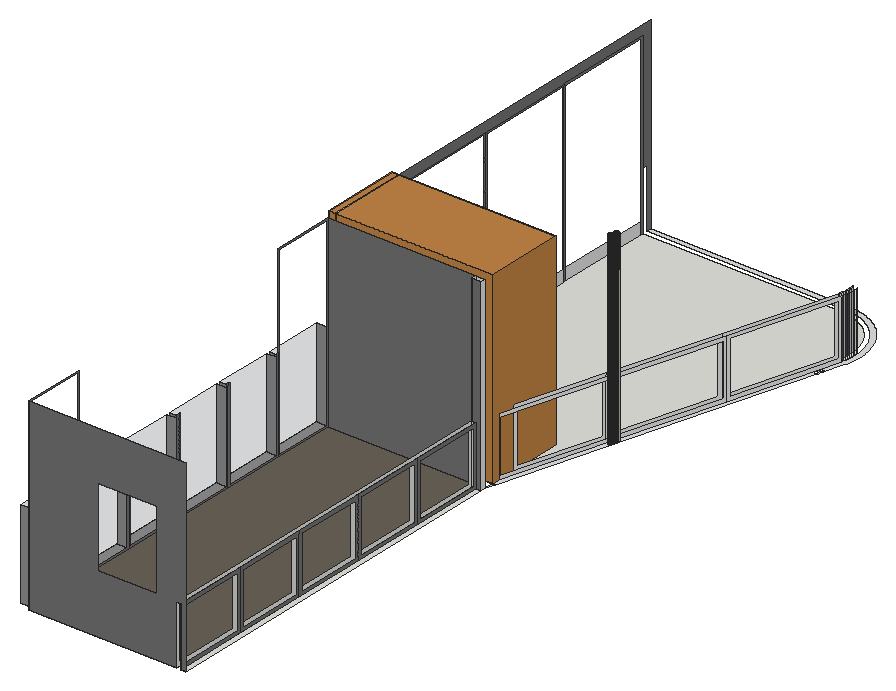
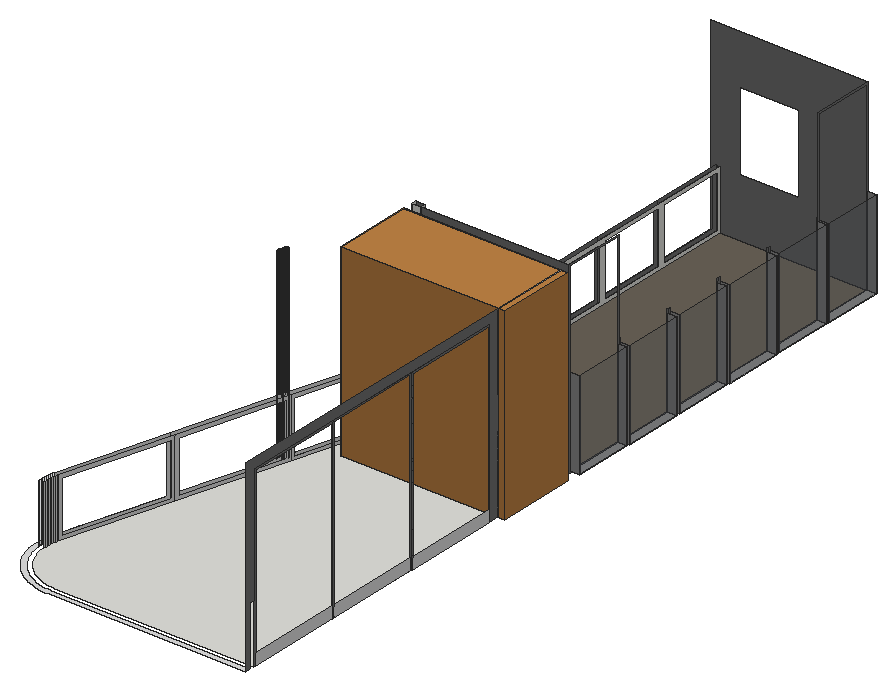
# SketchUp Ruby script. Lengths in inches.
U = 1.inch
M = Sketchup.active_model
def pt(a) = Geom::Point3d.new(a.map { |v| v * U })
def face(e, loops, mat)
  f = e.add_face(loops[0].map { |a| pt(a) })
  loops[1..].each { |l| e.add_face(l.map { |a| pt(a) }).erase! }
  f.material = f.back_material = mat if mat
  f
end
# faces: each face lists its corners as indices into pts; further lists are holes
def faces(e, pts, list, mat = nil) = list.each { |f| face(e, (f[0].is_a?(Array) ? f : [f]).map { |l| l.map { |i| pts[i] } }, mat) }
# xy, xz, yz: faces in a plane at the given z, y or x. An outline is a flat list of corners, or four numbers for a rectangle; further outlines are holes
def ring(l) = l.size == 4 ? [[l[0], l[1]], [l[2], l[1]], [l[2], l[3]], [l[0], l[3]]] : l.each_slice(2).to_a
def flat(e, list, mat, &to3) = list.each { |f| face(e, (f[0].is_a?(Array) ? f : [f]).map { |l| ring(l).map { |u, v| to3.(u, v) } }, mat) }
def xy(e, z, list, mat = nil) = flat(e, list, mat) { |x, y| [x, y, z] }
def xz(e, y, list, mat = nil) = flat(e, list, mat) { |x, z| [x, y, z] }
def yz(e, x, list, mat = nil) = flat(e, list, mat) { |y, z| [x, y, z] }
def lines(e, pts, list) = list.each { |a, b| e.add_line(pt(pts[a]), pt(pts[b])) }
# prism: a flat outline (further loops are holes) pulled along v
def prism(e, loops, v, mat = nil)
  f = face(e, loops, mat); d = Geom::Vector3d.new(v.map { |x| x * U })
  f.pushpull(f.normal.samedirection?(d) ? d.length : -d.length)
end
def box(e, o, s, mat = nil) = prism(e, [[o, [o[0] + s[0], o[1], o[2]], [o[0] + s[0], o[1] + s[1], o[2]], [o[0], o[1] + s[1], o[2]]]], [0, 0, s[2]], mat)
def at(x, y, z, deg = 0) = Geom::Transformation.translation(pt([x, y, z])) * Geom::Transformation.rotation(ORIGIN, Z_AXIS, deg.degrees)
def axes(o, x, y, z) = Geom::Transformation.new([*x, 0, *y, 0, *z, 0, *pt(o).to_a, 1])
def part(name) = M.definitions.add(name)
# library, detail: a bought-in or finely detailed component or shape, given as its bounding box
def library(name, o, s) = part(name).tap { |d| box(d.entities, o, s) }
def detail(e, o, s) = box(e.add_group.entities, o, s)
def put(e, d, t, mat = nil) = e.add_instance(d, t).tap { |i| i.material = mat if mat }
def group(e, t, mat = nil) = e.add_group.tap { |g| g.transformation = t; g.material = mat if mat }.entities
root = M.entities
M.materials.add("Glass_Basic_01").color = [105, 113, 122]
M.materials["Glass_Basic_01"].alpha = 0.25
M.materials.add("M01_Silver_Fog").color = [224, 224, 224]
M.materials.add("M04_Stone_Frost").color = [142, 142, 142]
M.materials.add("M06_Steel_Smoke").color = [114, 114, 114]
M.materials.add("Plaster_04_1K").color = [106, 98, 87]
M.materials.add("Wood_Floor_01_1K").color = [193, 132, 69]
c1 = part("Group\#1")
box(c1.entities,[-3.94,0,0],[99.94,48,114])
xy(root,396,[[303,6,306,231],[306,234,307.76,240,306,240],[216,246,303.26,246,306,255.36,321.22,307.35,340.07,371.78,359.17,437.01,359.4,437.91,359.63,439,359.83,440.1,359.98,441.21,360.09,442.32,360.16,443.43,360.1875,444.55,360.17,445.67,360.11,446.78,360.01,447.89,359.87,449,359.68,450.1,359.45,451.2,359.18,452.28,358.875,453.35,358.52,454.41,358.13,455.46,357.7,456.49,357.23,457.5,356.73,458.5,356.18,459.47,355.6,460.43,354.98,461.36,354.33,462.26,353.64,463.14,352.92,464,352.17,464.83,351.39,465.62,350.58,466.39,349.74,467.125,348.87,467.83,347.97,468.5,347.05,469.13,346.11,469.73,345.15,470.29,344.16,470.82,343.16,471.3,342.13,471.75,341.09,472.16,340.04,472.53,338.97,472.86,337.89,473.15,336.8,473.4,335.71,473.6,334.6,473.77,333.49,473.89,332.38,473.97,331.45,474,210,474,210,288,213,288,213,287.79,216,287.79]])
xy(root,396,[[[210,240,307.76,240,364.95,435.42,365.24,436.52,365.52,437.84,365.76,439.16,365.94,440.5,366.07,441.84,366.16,443.18,366.1875,444.52,366.17,445.87,366.1,447.21,365.98,448.55,365.8,449.89,365.58,451.21,365.3,452.53,364.98,453.84,364.61,455.13,364.18,456.41,363.71,457.67,363.2,458.91,362.63,460.13,362.02,461.33,361.36,462.5,360.69,463.59,360.66,463.65,359.92,464.77,359.13,465.86,358.3,466.92,357.4375,467.95,357.39,468,356.53,468.95,355.59,469.91,354.61,470.83,353.6,471.72,352.55,472.5625,351.47,473.37,350.37,474.13,349.23,474.85,348.07,475.53,346.88,476.16,345.67,476.75,344.44,477.29,343.1875,477.79,341.92,478.23,340.63,478.63,339.33,478.98,338.02,479.28,336.7,479.52,335.37,479.72,334.03,479.87,332.69,479.96,331.55,480,210,480,210,477,331.5,477,332.53,476.97,333.76,476.88,334.99,476.74,336.2,476.5625,337.41,476.34,338.61,476.0625,339.8,475.75,340.98,475.38,342.14,474.97,343.29,474.52,344.41,474.03,345.52,473.49,346.61,472.91,347.67,472.29,348.71,471.63,349.72,470.93,350.71,470.19,351.67,469.42,352.59,468.61,353.49,467.76,354.35,466.89,355.17,465.98,355.18,465.98,355.97,465.03,356.73,464.0625,357.45,463.0625,358.13,462.04,358.13,462.03,358.77,460.99,359.37,459.91,359.93,458.82,360.45,457.7,360.92,456.5625,361.35,455.41,361.74,454.24,362.08,453.06,362.38,451.86,362.63,450.66,362.83,449.44,362.99,448.22,363.1,447,363.17,445.77,363.1875,444.54,363.16,443.31,363.08,442.08,362.96,440.85,362.79,439.63,362.58,438.42,362.32,437.22,362.06,436.22,343.2,371.78,324.34,307.35,305.51,243,213,243,213,288,210,288],[358.91,418.8,358.82,418.81,358.73,418.8125,358.65,418.83,358.5625,418.85,358.48,418.87,358.39,418.9,358.3125,418.9375,358.24,418.98,358.16,419.02,358.09,419.07,357.95,419.18,357.89,419.24,357.83,419.31,357.73,419.45,357.68,419.53,357.64,419.61,357.61,419.6875,357.58,419.77,357.55,419.85,357.54,419.94,357.52,420.03,357.51,420.11,357.51,420.29,357.52,420.38,357.54,420.46,357.55,420.55,357.58,420.64,357.64,420.8,357.68,420.88,357.73,420.95,357.78,421.03,357.83,421.09,357.89,421.16,357.95,421.22,358.09,421.34,358.16,421.38,358.24,421.43,358.3125,421.47,358.39,421.5,358.48,421.53,358.5625,421.56,358.65,421.58,358.73,421.59,358.82,421.6,359,421.6,359.09,421.59,359.17,421.58,359.26,421.56,359.34,421.53,359.43,421.5,359.51,421.47,359.58,421.43,359.66,421.38,359.73,421.34,359.87,421.22,359.93,421.16,359.99,421.09,360.04,421.03,360.09,420.95,360.14,420.88,360.18,420.8,360.24,420.64,360.27,420.55,360.29,420.46,360.3,420.38,360.31,420.29,360.31,420.11,360.3,420.03,360.29,419.94,360.27,419.85,360.24,419.77,360.21,419.6875,360.18,419.61,360.14,419.53,360.09,419.45,359.99,419.31,359.93,419.24,359.87,419.18,359.73,419.07,359.66,419.02,359.58,418.98,359.51,418.9375,359.43,418.9,359.34,418.87,359.26,418.85,359.17,418.83,359.09,418.8125,359,418.81],[359.74,421.95,359.66,421.96,359.57,421.97,359.48,421.99,359.32,422.05,359.23,422.08,359.16,422.12,359.08,422.17,359.01,422.21,358.9375,422.27,358.87,422.33,358.75,422.45,358.7,422.52,358.65,422.6,358.6,422.67,358.5625,422.75,358.53,422.83,358.5,422.91,358.47,423,358.46,423.08,358.44,423.17,358.43,423.26,358.43,423.44,358.44,423.52,358.46,423.61,358.47,423.7,358.53,423.86,358.5625,423.94,358.6,424.02,358.65,424.1,358.75,424.24,358.81,424.31,358.87,424.37,358.9375,424.43,359.01,424.48,359.08,424.53,359.16,424.57,359.23,424.61,359.32,424.65,359.4,424.68,359.48,424.7,359.66,424.74,359.74,424.74,359.83,424.75,359.92,424.74,360.01,424.74,360.09,424.72,360.18,424.7,360.26,424.68,360.35,424.65,360.51,424.57,360.58,424.53,360.72,424.43,360.79,424.37,360.85,424.31,360.91,424.24,361.01,424.1,361.06,424.02,361.1,423.94,361.16,423.78,361.1875,423.7,361.21,423.61,361.22,423.52,361.23,423.44,361.23,423.26,361.21,423.08,361.1875,423,361.16,422.91,361.1,422.75,361.06,422.67,361.01,422.6,360.96,422.52,360.91,422.45,360.79,422.33,360.65,422.21,360.58,422.17,360.51,422.12,360.43,422.08,360.35,422.05,360.26,422.02,360.18,421.99,360.09,421.97,360.01,421.96,359.92,421.95],[325.27,304.17,325.18,304.18,325.09,304.1875,325.01,304.2,324.92,304.23,324.84,304.25,324.6,304.37,324.39,304.52,324.32,304.58,324.26,304.65,324.11,304.86,324.03,305.02,324,305.1,323.97,305.1875,323.95,305.27,323.9375,305.36,323.93,305.44,323.92,305.53,323.92,305.62,323.93,305.71,323.9375,305.8,323.96,305.88,323.98,305.97,324,306.05,324.12,306.29,324.27,306.5,324.33,306.56,324.4,306.625,324.47,306.68,324.61,306.78,324.77,306.86,324.85,306.89,324.9375,306.92,325.02,306.9375,325.11,306.95,325.2,306.96,325.28,306.97,325.37,306.97,325.55,306.95,325.63,306.93,325.72,306.91,325.88,306.85,325.96,306.8125,326.04,306.77,326.18,306.67,326.25,306.61,326.31,306.55,326.375,306.49,326.43,306.42,326.53,306.28,326.61,306.12,326.64,306.04,326.67,305.95,326.6875,305.87,326.7,305.78,326.71,305.69,326.72,305.61,326.72,305.52,326.7,305.34,326.68,305.26,326.66,305.17,326.6,305.01,326.5625,304.93,326.52,304.85,326.42,304.71,326.3,304.57,326.24,304.51,326.03,304.36,325.87,304.28,325.79,304.25,325.7,304.22,325.62,304.2,325.53,304.1875,325.44,304.17],[326.2,307.35,326.02,307.37,325.9375,307.38,325.85,307.41,325.77,307.43,325.6875,307.47,325.61,307.5,325.53,307.55,325.32,307.7,325.26,307.76,325.14,307.9,325.04,308.04,324.96,308.2,324.93,308.28,324.9,308.37,324.88,308.45,324.87,308.54,324.85,308.71,324.85,308.8,324.87,308.98,324.89,309.0625,324.91,309.15,324.9375,309.23,324.97,309.3125,325.01,309.39,325.05,309.47,325.2,309.68,325.27,309.74,325.33,309.8,325.4,309.86,325.54,309.96,325.7,310.04,325.78,310.07,325.87,310.1,325.95,310.12,326.04,310.13,326.21,310.15,326.3,310.15,326.48,310.13,326.5625,310.11,326.65,310.09,326.73,310.0625,326.8125,310.03,326.89,309.99,326.97,309.95,327.11,309.85,327.25,309.73,327.31,309.67,327.46,309.46,327.54,309.3,327.57,309.22,327.6,309.13,327.62,309.05,327.63,308.96,327.65,308.79,327.65,308.7,327.63,308.52,327.61,308.4375,327.59,308.35,327.56,308.27,327.53,308.1875,327.49,308.11,327.45,308.03,327.4,307.96,327.35,307.88,327.3,307.82,327.17,307.69,326.96,307.54,326.8,307.46,326.72,307.43,326.63,307.4,326.55,307.38,326.46,307.36,326.375,307.35]]],"M01_Silver_Fog")
xy(root,396,[[210,6,300,234]],"Plaster_04_1K")
xy(root,397,[[204,7,210,43],[204,45,210,81],[204,83,210,119],[204,121,210,157],[204,159,210,195],
  [204,197,210,233]],"M04_Stone_Frost")
xz(root,6,[[[210,396,210,510,306,510,306,396,303,396,303,432,300,432,300,396],[252,432,288,480]]],"M06_Steel_Smoke")
xz(root,7,[[204,397,210,451]],"M04_Stone_Frost")
xz(root,43,[[204,397,210,451]],"M04_Stone_Frost")
xz(root,45,[[204,397,210,451]],"M04_Stone_Frost")
xz(root,81,[[204,397,210,451]],"M04_Stone_Frost")
xz(root,83,[[204,397,210,451]],"M04_Stone_Frost")
xz(root,119,[[204,397,210,451]],"M04_Stone_Frost")
xz(root,121,[[204,397,210,451]],"M04_Stone_Frost")
xz(root,157,[[204,397,210,451]],"M04_Stone_Frost")
xz(root,159,[[204,397,210,451]],"M04_Stone_Frost")
xz(root,195,[[204,397,210,451]],"M04_Stone_Frost")
xz(root,197,[[204,397,210,451]],"M04_Stone_Frost")
xz(root,231,[[303,396,306,396,306,510,300,510,300,432,303,432]],"M06_Steel_Smoke")
xz(root,233,[[204,397,210,451]],"M04_Stone_Frost")
xz(root,234,[[300,396,306,510]])
xz(root,234,[[210,396,300,510]],"M06_Steel_Smoke")
xz(root,243,[[213,396,305.51,432]],"M01_Silver_Fog")
xz(root,246,[[216,396,303.26,432]],"M01_Silver_Fog")
xz(root,287.79,[[213,396,216,432]],"M01_Silver_Fog")
xz(root,304.17,[[325.27,396,325.36,510],[325.36,396,325.44,510]],"M01_Silver_Fog")
xz(root,306.97,[[325.28,396,325.37,510]],"M01_Silver_Fog")
xz(root,307.35,[[326.2,396,326.29,510],[326.29,396,326.375,510]],"M01_Silver_Fog")
xz(root,310.15,[[326.21,396,326.3,510]],"M01_Silver_Fog")
yz(root,204,[[7,397,43,451],[45,397,81,451],[83,397,119,451],[121,397,157,451],[159,397,195,451],
  [197,397,233,451]],"Glass_Basic_01")
yz(root,210,[[240,396,288,396,288,442.46,286.46,442.46,286.46,463.54,288,463.54,288,510,240,510]])
yz(root,210,[[295,396,353,403],[355,396,413,403],[415,396,473,403]],"M01_Silver_Fog")
yz(root,210,[[6,396,44,396,44,453,43,453,43,397,7,397,7,509,43,509,43,453,44,453,44,510,6,510],[44,396,82,396,82,453,81,453,81,397,45,397,45,453,44,453],[82,396,120,396,120,453,119,453,119,397,83,397,83,453,82,453],[120,396,158,396,158,453,157,453,157,397,121,397,121,453,120,453],[158,396,196,396,196,453,195,453,195,397,159,397,159,453,158,453],
  [196,396,234,396,234,510,196,510,196,453,197,453,197,509,233,509,233,397,197,397,197,453,196,453],[288,396,294,396,294,504,474,504,474,432,477,432,477,396,480,396,480,510,288,510],[294,396,295,396,295,503,353,503,353,396,354,396,354,504,294,504],[354,396,355,396,355,503,413,503,413,396,414,396,414,504,354,504],[414,396,415,396,415,503,473,503,473,396,474,396,474,504,414,504]],"M06_Steel_Smoke")
yz(root,213,[[243,396,287.79,432]],"M01_Silver_Fog")
yz(root,216,[[246,396,287.79,432]],"M01_Silver_Fog")
yz(root,300,[[[6,396,231,432],[8,398,49,430],[143,398,184,430],[188,398,229,430],[53,398,94,430],[98,398,139,430]],[231,396,234,510]])
yz(root,303,[[[6,396,51,432],[8,398,49,430]],[[51,396,96,432],[53,398,94,430]],[[96,396,141,432],[98,398,139,430]],[[141,396,186,432],[143,398,184,430]],[[186,396,231,432],[188,398,229,430]]],"M06_Steel_Smoke")
yz(root,306,[[231,396,234,510]])
yz(root,323.92,[[305.53,396,305.62,510]],"M01_Silver_Fog")
yz(root,324.85,[[308.71,396,308.8,510]],"M01_Silver_Fog")
yz(root,326.72,[[305.52,396,305.61,510]],"M01_Silver_Fog")
yz(root,327.65,[[308.7,396,308.79,510]],"M01_Silver_Fog")
p = [[305.51,243,396],[324.34,307.35,396],[324.34,307.35,432],[305.51,243,432],[323.78,305.43,430],[323.78,305.43,398],
  [306.07,244.92,398],[306.07,244.92,430],[303.26,246,432],[306,255.36,432],[306,255.36,396],[303.26,246,396],
  [321.22,307.35,432],[321.22,307.35,396],[320.65,305.43,430],[306.5625,257.28,430],[306.5625,257.28,398],[320.65,305.43,398],
  [324.84,304.25,396],[324.92,304.23,396],[324.92,304.23,510],[324.84,304.25,510],[325.01,304.2,396],[325.01,304.2,510],
  [325.09,304.1875,396],[325.09,304.1875,510],[325.18,304.18,396],[325.18,304.18,510],[325.27,304.17,396],[325.27,304.17,510],
  [325.44,304.17,396],[325.53,304.1875,396],[325.53,304.1875,510],[325.44,304.17,510],[325.62,304.2,396],[325.62,304.2,510],
  [325.7,304.22,396],[325.7,304.22,510],[325.79,304.25,396],[325.79,304.25,510],[325.87,304.28,396],[325.87,304.28,510],
  [324.6,304.37,396],[324.68,304.33,396],[324.68,304.33,510],[324.6,304.37,510],[324.76,304.29,396],[324.76,304.29,510],
  [325.95,304.32,396],[325.95,304.32,510],[326.03,304.36,396],[326.03,304.36,510],[324.53,304.42,396],[324.53,304.42,510],
  [324.46,304.47,396],[324.46,304.47,510],[326.1,304.41,396],[326.1,304.41,510],[326.17,304.46,396],[326.17,304.46,510],
  [324.32,304.58,396],[324.39,304.52,396],[324.39,304.52,510],[324.32,304.58,510],[326.24,304.51,396],[326.24,304.51,510],
  [326.3,304.57,396],[326.3,304.57,510],[324.21,304.72,396],[324.26,304.65,396],[324.26,304.65,510],[324.21,304.72,510],
  [326.36,304.64,396],[326.36,304.64,510],[326.42,304.71,396],[326.42,304.71,510],[324.16,304.79,396],[324.16,304.79,510],
  [326.47,304.78,396],[326.47,304.78,510],[324.11,304.86,396],[324.11,304.86,510],[326.52,304.85,396],[326.52,304.85,510],
  [324.03,305.02,396],[324.07,304.94,396],[324.07,304.94,510],[324.03,305.02,510],[326.5625,304.93,396],[326.5625,304.93,510],
  [326.6,305.01,396],[326.6,305.01,510],[324,305.1,396],[324,305.1,510],[326.63,305.09,396],[326.63,305.09,510],
  [323.97,305.1875,396],[323.97,305.1875,510],[326.66,305.17,396],[326.66,305.17,510],[323.95,305.27,396],[323.95,305.27,510],
  [326.68,305.26,396],[326.68,305.26,510],[323.9375,305.36,396],[323.9375,305.36,510],[326.7,305.34,396],[326.7,305.34,510],
  [326.71,305.43,396],[326.71,305.43,510],[323.93,305.44,396],[323.93,305.44,510],[323.92,305.53,396],[323.92,305.53,510],
  [326.72,305.52,396],[326.72,305.52,510],[323.93,305.71,396],[323.92,305.62,396],[323.92,305.62,510],[323.93,305.71,510],
  [326.72,305.61,396],[326.71,305.69,396],[326.71,305.69,510],[326.72,305.61,510],[323.9375,305.8,396],[323.9375,305.8,510],
  [326.7,305.78,396],[326.7,305.78,510],[323.96,305.88,396],[323.96,305.88,510],[326.6875,305.87,396],[326.6875,305.87,510],
  [323.98,305.97,396],[323.98,305.97,510],[326.67,305.95,396],[326.67,305.95,510],[324,306.05,396],[324,306.05,510],
  [326.64,306.04,396],[326.64,306.04,510],[326.61,306.12,396],[326.61,306.12,510],[324.04,306.13,396],[324.04,306.13,510],
  [324.08,306.21,396],[324.08,306.21,510],[326.57,306.2,396],[326.57,306.2,510],[324.12,306.29,396],[324.12,306.29,510],
  [326.53,306.28,396],[326.53,306.28,510],[324.17,306.36,396],[324.17,306.36,510],[326.48,306.35,396],[326.48,306.35,510],
  [324.22,306.43,396],[324.22,306.43,510],[324.27,306.5,396],[324.27,306.5,510],[326.43,306.42,396],[326.43,306.42,510],
  [326.375,306.49,396],[326.375,306.49,510],[324.33,306.56,396],[324.33,306.56,510],[326.31,306.55,396],[326.31,306.55,510],
  [324.4,306.625,396],[324.4,306.625,510],[324.47,306.68,396],[324.47,306.68,510],[326.25,306.61,396],[326.18,306.67,396],
  [326.18,306.67,510],[326.25,306.61,510],[324.54,306.73,396],[324.54,306.73,510],[324.61,306.78,396],[324.61,306.78,510],
  [326.11,306.72,396],[326.04,306.77,396],[326.04,306.77,510],[326.11,306.72,510],[324.69,306.82,396],[324.69,306.82,510],
  [324.77,306.86,396],[324.77,306.86,510],[325.96,306.8125,396],[325.88,306.85,396],[325.88,306.85,510],[325.96,306.8125,510],
  [324.85,306.89,396],[324.85,306.89,510],[324.9375,306.92,396],[324.9375,306.92,510],[325.02,306.9375,396],[325.02,306.9375,510],
  [325.11,306.95,396],[325.11,306.95,510],[325.63,306.93,396],[325.55,306.95,396],[325.55,306.95,510],[325.63,306.93,510],
  [325.72,306.91,396],[325.72,306.91,510],[325.8,306.88,396],[325.8,306.88,510],[325.2,306.96,396],[325.2,306.96,510],
  [325.28,306.97,396],[325.28,306.97,510],[325.46,306.96,396],[325.37,306.97,396],[325.37,306.97,510],[325.46,306.96,510],
  [340.07,371.78,432],[340.07,371.78,396],[339.51,369.86,398],[339.51,369.86,430],[321.78,309.27,430],[321.78,309.27,398],
  [343.2,371.78,432],[343.2,371.78,396],[324.9,309.27,398],[324.9,309.27,430],[342.64,369.86,430],[342.64,369.86,398],
  [326.11,307.36,396],[326.2,307.35,396],[326.2,307.35,510],[326.11,307.36,510],[325.6875,307.47,396],[325.77,307.43,396],
  [325.77,307.43,510],[325.6875,307.47,510],[325.85,307.41,396],[325.85,307.41,510],[325.9375,307.38,396],[326.02,307.37,396],
  [326.02,307.37,510],[325.9375,307.38,510],[326.375,307.35,396],[326.46,307.36,396],[326.46,307.36,510],[326.375,307.35,510],
  [326.55,307.38,396],[326.55,307.38,510],[326.63,307.4,396],[326.63,307.4,510],[326.72,307.43,396],[326.72,307.43,510],
  [326.8,307.46,396],[326.8,307.46,510],[325.53,307.55,396],[325.61,307.5,396],[325.61,307.5,510],[325.53,307.55,510],
  [325.46,307.6,396],[325.46,307.6,510],[326.88,307.5,396],[326.88,307.5,510],[326.96,307.54,396],[326.96,307.54,510],
  [327.03,307.59,396],[327.03,307.59,510],[325.32,307.7,396],[325.39,307.65,396],[325.39,307.65,510],[325.32,307.7,510],
  [327.1,307.64,396],[327.1,307.64,510],[327.17,307.69,396],[327.17,307.69,510],[325.26,307.76,396],[325.26,307.76,510],
  [327.23,307.75,396],[327.23,307.75,510],[325.14,307.9,396],[325.2,307.83,396],[325.2,307.83,510],[325.14,307.9,510],
  [327.3,307.82,396],[327.3,307.82,510],[327.35,307.88,396],[327.35,307.88,510],[325.09,307.97,396],[325.09,307.97,510],
  [327.4,307.96,396],[327.4,307.96,510],[325.04,308.04,396],[325.04,308.04,510],[325,308.12,396],[325,308.12,510],
  [327.45,308.03,396],[327.45,308.03,510],[327.49,308.11,396],[327.49,308.11,510],[324.96,308.2,396],[324.96,308.2,510],
  [327.53,308.1875,396],[327.53,308.1875,510],[324.93,308.28,396],[324.93,308.28,510],[327.56,308.27,396],[327.56,308.27,510],
  [324.9,308.37,396],[324.9,308.37,510],[327.59,308.35,396],[327.59,308.35,510],[324.88,308.45,396],[324.88,308.45,510],
  [327.61,308.4375,396],[327.61,308.4375,510],[327.63,308.52,396],[327.63,308.52,510],[324.87,308.54,396],[324.87,308.54,510],
  [324.86,308.625,396],[324.86,308.625,510],[327.64,308.61,396],[327.64,308.61,510],[324.85,308.71,396],[324.85,308.71,510],
  [327.65,308.7,396],[327.65,308.7,510],[324.86,308.89,396],[324.85,308.8,396],[324.85,308.8,510],[324.86,308.89,510],
  [327.65,308.79,396],[327.64,308.875,396],[327.64,308.875,510],[327.65,308.79,510],[324.87,308.98,396],[324.87,308.98,510],
  [327.63,308.96,396],[327.63,308.96,510],[324.89,309.0625,396],[324.89,309.0625,510],[327.62,309.05,396],[327.62,309.05,510],
  [327.6,309.13,396],[327.6,309.13,510],[324.91,309.15,396],[324.91,309.15,510],[324.9375,309.23,396],[324.9375,309.23,510],
  [327.57,309.22,396],[327.57,309.22,510],[324.97,309.3125,396],[324.97,309.3125,510],[327.54,309.3,396],[327.54,309.3,510],
  [325.01,309.39,396],[325.01,309.39,510],[327.5,309.38,396],[327.5,309.38,510],[325.05,309.47,396],[325.05,309.47,510],
  [327.46,309.46,396],[327.46,309.46,510],[325.1,309.54,396],[325.1,309.54,510],[325.15,309.61,396],[325.15,309.61,510],
  [327.41,309.53,396],[327.41,309.53,510],[327.36,309.6,396],[327.36,309.6,510],[325.2,309.68,396],[325.2,309.68,510],
  [327.31,309.67,396],[327.31,309.67,510],[325.27,309.74,396],[325.27,309.74,510],[325.33,309.8,396],[325.33,309.8,510],
  [327.25,309.73,396],[327.25,309.73,510],[327.18,309.79,396],[327.18,309.79,510],[325.4,309.86,396],[325.4,309.86,510],
  [327.11,309.85,396],[327.11,309.85,510],[325.47,309.91,396],[325.47,309.91,510],[325.54,309.96,396],[325.54,309.96,510],
  [327.04,309.9,396],[327.04,309.9,510],[326.97,309.95,396],[326.97,309.95,510],[325.62,310,396],[325.62,310,510],
  [325.7,310.04,396],[325.7,310.04,510],[325.78,310.07,396],[325.78,310.07,510],[326.8125,310.03,396],[326.73,310.0625,396],
  [326.73,310.0625,510],[326.8125,310.03,510],[326.89,309.99,396],[326.89,309.99,510],[325.87,310.1,396],[325.87,310.1,510],
  [325.95,310.12,396],[325.95,310.12,510],[326.04,310.13,396],[326.04,310.13,510],[326.125,310.14,396],[326.125,310.14,510],
  [326.21,310.15,396],[326.21,310.15,510],[326.39,310.14,396],[326.3,310.15,396],[326.3,310.15,510],[326.39,310.14,510],
  [326.48,310.13,396],[326.48,310.13,510],[326.5625,310.11,396],[326.5625,310.11,510],[326.65,310.09,396],[326.65,310.09,510],
  [359.17,437.01,396],[359.17,437.01,432],[340.64,373.7,398],[358.6,435.09,398],[358.6,435.09,430],[340.64,373.7,430],
  [362.06,436.22,432],[362.06,436.22,396],[343.76,373.7,430],[361.5,434.3,430],[361.5,434.3,398],[343.76,373.7,398],
  [362.32,437.22,396],[362.32,437.22,432],[359.4,437.91,396],[359.4,437.91,432],[362.58,438.42,396],[362.58,438.42,432],
  [359.63,439,396],[359.63,439,432],[362.79,439.63,396],[362.79,439.63,432],[359.83,440.1,396],[359.83,440.1,432],
  [362.96,440.85,396],[362.96,440.85,432],[359.98,441.21,396],[359.98,441.21,432],[363.08,442.08,396],[363.08,442.08,432],
  [360.09,442.32,396],[360.09,442.32,432],[363.16,443.31,396],[363.16,443.31,432],[360.16,443.43,396],[360.16,443.43,432],
  [363.1875,444.54,396],[363.1875,444.54,432],[360.1875,444.55,396],[360.1875,444.55,432],[360.17,445.67,396],[360.17,445.67,432],
  [363.17,445.77,396],[363.17,445.77,432],[360.11,446.78,396],[360.11,446.78,432],[363.1,447,396],[363.1,447,432],
  [209.78,288,510],[209.78,288,396],[305.48,242.91,396],[305.48,242.91,432]]
faces(root,p,[[[0,1,2,3],[4,5,6,7]],[8,9,10,11],[[9,12,13,10],[14,15,16,17]],[18,19,20,21],[19,22,23,20],[22,24,25,23],[24,26,27,25],[26,28,29,27],
  [30,31,32,33],[31,34,35,32],[34,36,37,35],[36,38,39,37],[38,40,41,39],[42,43,44,45],[43,46,47,44],[46,18,21,47],
  [40,48,49,41],[48,50,51,49],[52,42,45,53],[54,52,53,55],[50,56,57,51],[56,58,59,57],[60,61,62,63],[61,54,55,62],
  [58,64,65,59],[64,66,67,65],[68,69,70,71],[69,60,63,70],[66,72,73,67],[72,74,75,73],[76,68,71,77],[74,78,79,75],
  [80,76,77,81],[78,82,83,79],[84,85,86,87],[85,80,81,86],[82,88,89,83],[88,90,91,89],[92,84,87,93],[90,94,95,91],
  [96,92,93,97],[94,98,99,95],[100,96,97,101],[98,102,103,99],[104,100,101,105],[102,106,107,103],[106,108,109,107],[110,104,105,111],
  [112,110,111,113],[108,114,115,109],[116,117,118,119],[120,121,122,123],[124,116,119,125],[121,126,127,122],[128,124,125,129],[126,130,131,127],
  [132,128,129,133],[130,134,135,131],[136,132,133,137],[134,138,139,135],[138,140,141,139],[142,136,137,143],[144,142,143,145],[140,146,147,141],
  [148,144,145,149],[146,150,151,147],[152,148,149,153],[150,154,155,151],[156,152,153,157],[158,156,157,159],[154,160,161,155],[160,162,163,161],
  [164,158,159,165],[162,166,167,163],[168,164,165,169],[170,168,169,171],[172,173,174,175],[166,172,175,167],[176,170,171,177],[178,176,177,179],
  [180,181,182,183],[173,180,183,174],[184,178,179,185],[186,184,185,187],[188,189,190,191],[181,188,191,182],[192,186,187,193],[194,192,193,195],
  [196,194,195,197],[198,196,197,199],[200,201,202,203],[204,200,203,205],[206,204,205,207],[189,206,207,190],[208,198,199,209],[210,208,209,211],
  [212,213,214,215],[201,212,215,202],[[12,216,217,13],[218,219,220,221]],[[222,2,1,223],[224,225,226,227]],[228,229,230,231],[232,233,234,235],[233,236,237,234],[238,239,240,241],
  [236,238,241,237],[239,228,231,240],[242,243,244,245],[243,246,247,244],[246,248,249,247],[248,250,251,249],[250,252,253,251],[254,255,256,257],
  [258,254,257,259],[255,232,235,256],[252,260,261,253],[260,262,263,261],[262,264,265,263],[266,267,268,269],[267,258,259,268],[264,270,271,265],
  [270,272,273,271],[274,266,269,275],[272,276,277,273],[278,279,280,281],[279,274,275,280],[276,282,283,277],[282,284,285,283],[286,278,281,287],
  [284,288,289,285],[290,286,287,291],[292,290,291,293],[288,294,295,289],[294,296,297,295],[298,292,293,299],[296,300,301,297],[302,298,299,303],
  [300,304,305,301],[306,302,303,307],[304,308,309,305],[310,306,307,311],[308,312,313,309],[312,314,315,313],[316,310,311,317],[318,316,317,319],
  [314,320,321,315],[322,318,319,323],[320,324,325,321],[326,327,328,329],[330,331,332,333],[334,326,329,335],[331,336,337,332],[338,334,335,339],
  [336,340,341,337],[340,342,343,341],[344,338,339,345],[346,344,345,347],[342,348,349,343],[350,346,347,351],[348,352,353,349],[354,350,351,355],
  [352,356,357,353],[358,354,355,359],[356,360,361,357],[362,358,359,363],[364,362,363,365],[360,366,367,361],[366,368,369,367],[370,364,365,371],
  [368,372,373,369],[374,370,371,375],[376,374,375,377],[372,378,379,373],[378,380,381,379],[382,376,377,383],[380,384,385,381],[386,382,383,387],
  [388,386,387,389],[384,390,391,385],[390,392,393,391],[394,388,389,395],[396,394,395,397],[398,396,397,399],[400,401,402,403],[404,400,403,405],
  [392,404,405,393],[406,398,399,407],[408,406,407,409],[410,408,409,411],[412,410,411,413],[414,412,413,415],[416,417,418,419],[420,416,419,421],
  [422,420,421,423],[401,424,425,402],[424,422,423,425],[[426,217,216,427],[428,429,430,431]],[[432,222,223,433],[434,435,436,437]],[440,426,427,441],[444,440,441,445],[448,444,445,449],
  [452,448,449,453],[456,452,453,457],[460,456,457,461],[464,460,461,465],[466,464,465,467],[470,466,467,471]],"M01_Silver_Fog")
faces(root,p,[[433,438,439,432],[438,442,443,439],[442,446,447,443],[446,450,451,447],[450,454,455,451],[454,458,459,455],[458,462,463,459],[462,468,469,463],
  [468,472,473,469]],"Glass_Basic_01")
lines(root,p,[[474,475],[476,477]])
put(root,c1,at(210,240,396),"Wood_Floor_01_1K")
